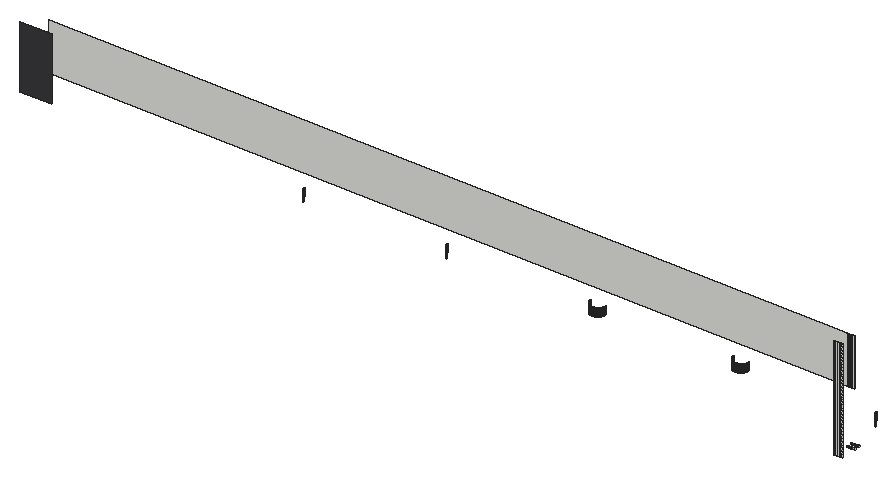
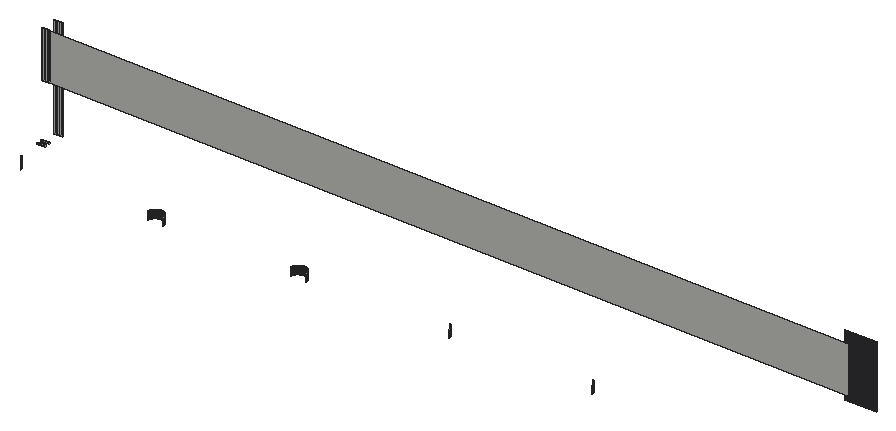
# SketchUp Ruby script. Lengths in inches.
U = 1.inch
M = Sketchup.active_model
def pt(a) = Geom::Point3d.new(a.map { |v| v * U })
def face(e, loops, mat)
  f = e.add_face(loops[0].map { |a| pt(a) })
  loops[1..].each { |l| e.add_face(l.map { |a| pt(a) }).erase! }
  f.material = f.back_material = mat if mat
  f
end
# faces: each face lists its corners as indices into pts; further lists are holes
def faces(e, pts, list, mat = nil) = list.each { |f| face(e, (f[0].is_a?(Array) ? f : [f]).map { |l| l.map { |i| pts[i] } }, mat) }
# xy, xz, yz: faces in a plane at the given z, y or x. An outline is a flat list of corners, or four numbers for a rectangle; further outlines are holes
def ring(l) = l.size == 4 ? [[l[0], l[1]], [l[2], l[1]], [l[2], l[3]], [l[0], l[3]]] : l.each_slice(2).to_a
def flat(e, list, mat, &to3) = list.each { |f| face(e, (f[0].is_a?(Array) ? f : [f]).map { |l| ring(l).map { |u, v| to3.(u, v) } }, mat) }
def xy(e, z, list, mat = nil) = flat(e, list, mat) { |x, y| [x, y, z] }
def xz(e, y, list, mat = nil) = flat(e, list, mat) { |x, z| [x, y, z] }
def yz(e, x, list, mat = nil) = flat(e, list, mat) { |y, z| [x, y, z] }
def lines(e, pts, list) = list.each { |a, b| e.add_line(pt(pts[a]), pt(pts[b])) }
# prism: a flat outline (further loops are holes) pulled along v
def prism(e, loops, v, mat = nil)
  f = face(e, loops, mat); d = Geom::Vector3d.new(v.map { |x| x * U })
  f.pushpull(f.normal.samedirection?(d) ? d.length : -d.length)
end
def box(e, o, s, mat = nil) = prism(e, [[o, [o[0] + s[0], o[1], o[2]], [o[0] + s[0], o[1] + s[1], o[2]], [o[0], o[1] + s[1], o[2]]]], [0, 0, s[2]], mat)
def at(x, y, z, deg = 0) = Geom::Transformation.translation(pt([x, y, z])) * Geom::Transformation.rotation(ORIGIN, Z_AXIS, deg.degrees)
def axes(o, x, y, z) = Geom::Transformation.new([*x, 0, *y, 0, *z, 0, *pt(o).to_a, 1])
def part(name) = M.definitions.add(name)
# library, detail: a bought-in or finely detailed component or shape, given as its bounding box
def library(name, o, s) = part(name).tap { |d| box(d.entities, o, s) }
def detail(e, o, s) = box(e.add_group.entities, o, s)
def put(e, d, t, mat = nil) = e.add_instance(d, t).tap { |i| i.material = mat if mat }
def group(e, t, mat = nil) = e.add_group.tap { |g| g.transformation = t; g.material = mat if mat }.entities
root = M.entities
M.materials.add("1432 AP 8245 TAR ROAD").color = [57, 57, 60]
xz(root,164,[[324,231,324.3125,270]])
xz(root,164,[[12,246,24,270]],"1432 AP 8245 TAR ROAD")
xz(root,170,[[324,231,324.24,231.5],[18,252,324,270],[324,252,324.24,270]])
xz(root,170.01,[[324.47,231,324.71,231.5],[324.47,252,324.71,270]])
xz(root,172,[[324,231,324.21,231.5]])
xz(root,172.01,[[324.42,231,324.63,231.5]])
xz(root,185,[[214.28,231,214.35,234],[214.35,231,214.43,234],[214.43,231,214.51,234],[269.08,231,269.15,234],[269.15,231,269.23,234],
  [269.23,231,269.3125,234]])
xz(root,185.01,[[214.12,231,214.2,234],[214.59,231,214.67,234],[268.92,231,269,234],[269.39,231,269.47,234]])
yz(root,156.61,[[187.73,231,187.81,234]])
yz(root,211.41,[[187.73,231,187.81,234]])
yz(root,217.39,[[187.72,231,187.8,234]])
yz(root,266.21,[[187.73,231,187.81,234]])
yz(root,321.01,[[187.73,231,187.81,234]])
p = [[324.63,164.01,231],[324.63,164.01,270],[324.3125,164,270],[324.3125,164,231],[324.94,164.02,231],[324.94,164.02,270],
  [325.26,164.03,231],[325.26,164.03,270],[325.57,164.05,231],[325.57,164.05,270],[325.88,164.07,231],[325.88,164.07,270],
  [326.2,164.1,231],[326.2,164.1,270],[326.51,164.13,231],[326.51,164.13,270],[326.82,164.17,231],[326.82,164.17,270],
  [327.13,164.21,231],[327.13,164.21,270],[324.47,170.01,231],[324.24,170,231],[324.24,170,231.5],[324.47,170.01,231.5],
  [324.94,170.02,231],[324.71,170.01,231],[324.71,170.01,231.5],[324.94,170.02,231.5],[325.18,170.04,231],[325.18,170.04,231.5],
  [325.41,170.06,231],[325.41,170.06,231.5],[325.65,170.08,231],[325.65,170.08,231.5],[325.88,170.1,231],[325.88,170.1,231.5],
  [326.12,170.125,231],[326.12,170.125,231.5],[326.35,170.15,231],[326.35,170.15,231.5],[326.58,170.1875,231],[326.58,170.1875,231.5],
  [326.82,170.22,231],[326.82,170.22,231.5],[327.05,170.26,231],[327.05,170.26,231.5],[327.28,170.3,231],[327.28,170.3,231.5],
  [324.21,172,231],[324.42,172.01,231],[324.42,172.01,231.5],[324.21,172,231.5],[324.63,172.01,231],[324.84,172.02,231],
  [324.84,172.02,231.5],[324.63,172.01,231.5],[325.05,172.03,231],[325.05,172.03,231.5],[325.26,172.05,231],[325.26,172.05,231.5],
  [325.46,172.07,231],[325.46,172.07,231.5],[325.67,172.09,231],[325.67,172.09,231.5],[325.88,172.11,231],[325.88,172.11,231.5],
  [326.09,172.14,231],[326.09,172.14,231.5],[326.3,172.17,231],[326.3,172.17,231.5],[326.5,172.2,231],[326.5,172.2,231.5],
  [326.71,172.23,231],[326.71,172.23,231.5],[326.92,172.27,231],[326.92,172.27,231.5],[327.12,172.31,231],[327.12,172.31,231.5],
  [213.89,185.04,231],[213.81,185.06,231],[213.81,185.06,234],[213.89,185.04,234],[213.96,185.03,231],[213.96,185.03,234],
  [214.04,185.02,231],[214.04,185.02,234],[214.12,185.01,231],[214.12,185.01,234],[214.28,185,231],[214.2,185.01,231],
  [214.2,185.01,234],[214.28,185,234],[214.59,185.01,231],[214.51,185,231],[214.51,185,234],[214.59,185.01,234],
  [214.75,185.02,231],[214.67,185.01,231],[214.67,185.01,234],[214.75,185.02,234],[214.82,185.03,231],[214.82,185.03,234],
  [214.9,185.04,231],[214.9,185.04,234],[214.98,185.06,231],[214.98,185.06,234],[268.6875,185.04,231],[268.61,185.06,231],
  [268.61,185.06,234],[268.6875,185.04,234],[268.76,185.03,231],[268.76,185.03,234],[268.84,185.02,231],[268.84,185.02,234],
  [268.92,185.01,231],[268.92,185.01,234],[269.08,185,231],[269,185.01,231],[269,185.01,234],[269.08,185,234],
  [269.39,185.01,231],[269.3125,185,231],[269.3125,185,234],[269.39,185.01,234],[269.55,185.02,231],[269.47,185.01,231],
  [269.47,185.01,234],[269.55,185.02,234],[269.625,185.03,231],[269.625,185.03,234],[269.7,185.04,231],[269.7,185.04,234],
  [269.78,185.06,231],[269.78,185.06,234],[103.9,185.14,231],[103.83,185.16,231],[103.83,185.16,234],[103.9,185.14,234],
  [158.7,185.14,231],[158.63,185.16,231],[158.63,185.16,234],[158.7,185.14,234],[213.5,185.14,231],[213.43,185.16,231],
  [213.43,185.16,234],[213.5,185.14,234],[213.58,185.11,231],[213.58,185.11,234],[213.66,185.09,231],[213.66,185.09,234],
  [213.73,185.08,231],[213.73,185.08,234],[215.06,185.07,231],[215.06,185.07,234],[215.13,185.09,231],[215.13,185.09,234],
  [215.21,185.11,231],[215.21,185.11,234],[215.28,185.13,231],[215.28,185.13,234],[215.36,185.16,231],[215.36,185.16,234],
  [268.3,185.14,231],[268.23,185.16,231],[268.23,185.16,234],[268.3,185.14,234],[268.38,185.11,231],[268.38,185.11,234],
  [268.46,185.09,231],[268.46,185.09,234],[268.53,185.08,231],[268.53,185.08,234],[269.86,185.07,231],[269.86,185.07,234],
  [269.93,185.09,231],[269.93,185.09,234],[270.01,185.11,231],[270.01,185.11,234],[270.08,185.13,231],[270.08,185.13,234],
  [270.16,185.16,231],[270.16,185.16,234],[323.1,185.14,231],[323.03,185.16,231],[323.03,185.16,234],[323.1,185.14,234],
  [103.61,185.25,231],[103.54,185.28,231],[103.54,185.28,234],[103.61,185.25,234],[103.68,185.22,231],[103.68,185.22,234],
  [103.76,185.1875,231],[103.76,185.1875,234],[158.41,185.25,231],[158.34,185.28,231],[158.34,185.28,234],[158.41,185.25,234],
  [158.48,185.22,231],[158.48,185.22,234],[158.56,185.1875,231],[158.56,185.1875,234],[213.21,185.25,231],[213.14,185.28,231],
  [213.14,185.28,234],[213.21,185.25,234],[213.28,185.22,231],[213.28,185.22,234],[213.36,185.1875,231],[213.36,185.1875,234],
  [215.43,185.18,231],[215.43,185.18,234],[215.51,185.21,231],[215.51,185.21,234],[215.58,185.24,231],[215.58,185.24,234],
  [215.65,185.27,231],[215.65,185.27,234],[268.01,185.25,231],[267.9375,185.28,231],[267.9375,185.28,234],[268.01,185.25,234],
  [268.08,185.22,231],[268.08,185.22,234],[268.16,185.1875,231],[268.16,185.1875,234],[270.23,185.18,231],[270.23,185.18,234],
  [270.31,185.21,231],[270.31,185.21,234],[270.38,185.24,231],[270.38,185.24,234],[270.45,185.27,231],[270.45,185.27,234],
  [322.81,185.25,231],[322.74,185.28,231],[322.74,185.28,234],[322.81,185.25,234],[322.88,185.22,231],[322.88,185.22,234],
  [322.96,185.1875,231],[322.96,185.1875,234],[103.4,185.35,231],[103.33,185.39,231],[103.33,185.39,234],[103.4,185.35,234],
  [103.47,185.3125,231],[103.47,185.3125,234],[158.2,185.35,231],[158.13,185.39,231],[158.13,185.39,234],[158.2,185.35,234],
  [158.27,185.3125,231],[158.27,185.3125,234],[213,185.35,231],[212.93,185.39,231],[212.93,185.39,234],[213,185.35,234],
  [213.07,185.3125,231],[213.07,185.3125,234],[215.72,185.31,231],[215.72,185.31,234],[215.79,185.34,231],[215.79,185.34,234],
  [215.86,185.38,231],[215.86,185.38,234],[267.8,185.35,231],[267.73,185.39,231],[267.73,185.39,234],[267.8,185.35,234],
  [267.87,185.3125,231],[267.87,185.3125,234],[270.52,185.31,231],[270.52,185.31,234],[270.59,185.34,231],[270.59,185.34,234],
  [270.66,185.38,231],[270.66,185.38,234],[322.6,185.35,231],[322.53,185.39,231],[322.53,185.39,234],[322.6,185.35,234],
  [322.67,185.3125,231],[322.67,185.3125,234],[103.26,185.42,231],[103.19,185.47,231],[103.19,185.47,234],[103.26,185.42,234],
  [158.0625,185.42,231],[157.99,185.47,231],[157.99,185.47,234],[158.0625,185.42,234],[212.86,185.42,231],[212.79,185.47,231],
  [212.79,185.47,234],[212.86,185.42,234],[215.93,185.42,231],[215.93,185.42,234],[216,185.46,231],[216,185.46,234],
  [267.66,185.42,231],[267.59,185.47,231],[267.59,185.47,234],[267.66,185.42,234],[270.73,185.42,231],[270.73,185.42,234],
  [270.8,185.46,231],[270.8,185.46,234],[322.46,185.42,231],[322.39,185.47,231],[322.39,185.47,234],[322.46,185.42,234],
  [103.13,185.51,231],[103.0625,185.55,231],[103.0625,185.55,234],[103.13,185.51,234],[157.93,185.51,231],[157.86,185.55,231],
  [157.86,185.55,234],[157.93,185.51,234],[212.73,185.51,231],[212.66,185.55,231],[212.66,185.55,234],[212.73,185.51,234],
  [216.0625,185.5,231],[216.0625,185.5,234],[216.125,185.55,231],[216.125,185.55,234],[216.19,185.59,231],[216.19,185.59,234],
  [267.53,185.51,231],[267.46,185.55,231],[267.46,185.55,234],[267.53,185.51,234],[270.86,185.5,231],[270.86,185.5,234],
  [270.93,185.55,231],[270.93,185.55,234],[270.99,185.59,231],[270.99,185.59,234],[322.33,185.51,231],[322.26,185.55,231],
  [322.26,185.55,234],[322.33,185.51,234],[102.9375,185.65,231],[102.88,185.7,231],[102.88,185.7,234],[102.9375,185.65,234],
  [103,185.6,231],[103,185.6,234],[157.74,185.65,231],[157.68,185.7,231],[157.68,185.7,234],[157.74,185.65,234],
  [157.8,185.6,231],[157.8,185.6,234],[212.54,185.65,231],[212.48,185.7,231],[212.48,185.7,234],[212.54,185.65,234],
  [212.6,185.6,231],[212.6,185.6,234],[216.25,185.64,231],[216.25,185.64,234],[216.3125,185.69,231],[216.3125,185.69,234],
  [267.34,185.65,231],[267.28,185.7,231],[267.28,185.7,234],[267.34,185.65,234],[267.4,185.6,231],[267.4,185.6,234],
  [271.05,185.64,231],[271.05,185.64,234],[271.11,185.69,231],[271.11,185.69,234],[322.14,185.65,231],[322.08,185.7,231],
  [322.08,185.7,234],[322.14,185.65,234],[322.2,185.6,231],[322.2,185.6,234],[102.82,185.75,231],[102.76,185.8,231],
  [102.76,185.8,234],[102.82,185.75,234],[157.62,185.75,231],[157.56,185.8,231],[157.56,185.8,234],[157.62,185.75,234],
  [212.42,185.75,231],[212.36,185.8,231],[212.36,185.8,234],[212.42,185.75,234],[216.375,185.74,231],[216.375,185.74,234],
  [216.43,185.79,231],[216.43,185.79,234],[267.22,185.75,231],[267.16,185.8,231],[267.16,185.8,234],[267.22,185.75,234],
  [271.17,185.74,231],[271.17,185.74,234],[271.23,185.79,231],[271.23,185.79,234],[322.02,185.75,231],[321.96,185.8,231],
  [321.96,185.8,234],[322.02,185.75,234],[102.7,185.86,231],[102.7,185.86,234],[157.5,185.86,231],[157.5,185.86,234],
  [212.3,185.86,231],[212.3,185.86,234],[216.49,185.85,231],[216.49,185.85,234],[216.54,185.9,231],[216.54,185.9,234],
  [267.1,185.86,231],[267.1,185.86,234],[271.29,185.85,231],[271.29,185.85,234],[271.34,185.9,231],[271.34,185.9,234],
  [321.9,185.86,231],[321.9,185.86,234],[102.65,185.91,231],[102.59,185.97,231],[102.59,185.97,234],[102.65,185.91,234],
  [157.45,185.91,231],[157.39,185.97,231],[157.39,185.97,234],[157.45,185.91,234],[212.25,185.91,231],[212.19,185.97,231],
  [212.19,185.97,234],[212.25,185.91,234],[216.6,185.96,231],[216.6,185.96,234],[267.05,185.91,231],[266.99,185.97,231],
  [266.99,185.97,234],[267.05,185.91,234],[271.4,185.96,231],[271.4,185.96,234],[321.85,185.91,231],[321.79,185.97,231],
  [321.79,185.97,234],[321.85,185.91,234],[102.54,186.03,231],[102.49,186.09,231],[102.49,186.09,234],[102.54,186.03,234],
  [157.34,186.03,231],[157.29,186.09,231],[157.29,186.09,234],[157.34,186.03,234],[212.14,186.03,231],[212.09,186.09,231],
  [212.09,186.09,234],[212.14,186.03,234],[216.65,186.02,231],[216.65,186.02,234],[216.7,186.08,231],[216.7,186.08,234],
  [266.94,186.03,231],[266.89,186.09,231],[266.89,186.09,234],[266.94,186.03,234],[271.45,186.02,231],[271.45,186.02,234],
  [271.5,186.08,231],[271.5,186.08,234],[321.74,186.03,231],[321.69,186.09,231],[321.69,186.09,234],[321.74,186.03,234],
  [102.44,186.15,231],[102.39,186.21,231],[102.39,186.21,234],[102.44,186.15,234],[157.24,186.15,231],[157.19,186.21,231],
  [157.19,186.21,234],[157.24,186.15,234],[212.04,186.15,231],[211.99,186.21,231],[211.99,186.21,234],[212.04,186.15,234],
  [216.75,186.14,231],[216.75,186.14,234],[216.8,186.2,231],[216.8,186.2,234],[266.84,186.15,231],[266.79,186.21,231],
  [266.79,186.21,234],[266.84,186.15,234],[271.55,186.14,231],[271.55,186.14,234],[271.6,186.2,231],[271.6,186.2,234],
  [321.64,186.15,231],[321.59,186.21,231],[321.59,186.21,234],[321.64,186.15,234],[102.35,186.27,231],[102.35,186.27,234],
  [157.15,186.27,231],[157.15,186.27,234],[211.95,186.27,231],[211.95,186.27,234],[216.85,186.26,231],[216.85,186.26,234],
  [266.75,186.27,231],[266.75,186.27,234],[271.65,186.26,231],[271.65,186.26,234],[321.55,186.27,231],[321.55,186.27,234],
  [102.3,186.34,231],[102.26,186.4,231],[102.26,186.4,234],[102.3,186.34,234],[157.1,186.34,231],[157.06,186.4,231],
  [157.06,186.4,234],[157.1,186.34,234],[211.9,186.34,231],[211.86,186.4,231],[211.86,186.4,234],[211.9,186.34,234],
  [216.89,186.33,231],[216.89,186.33,234],[216.93,186.39,231],[216.93,186.39,234],[266.7,186.34,231],[266.66,186.4,231],
  [266.66,186.4,234],[266.7,186.34,234],[271.69,186.33,231],[271.69,186.33,234],[271.73,186.39,231],[271.73,186.39,234],
  [321.5,186.34,231],[321.46,186.4,231],[321.46,186.4,234],[321.5,186.34,234],[102.22,186.47,231],[102.22,186.47,234],
  [157.02,186.47,231],[157.02,186.47,234],[211.82,186.47,231],[211.82,186.47,234],[216.98,186.46,231],[216.98,186.46,234],
  [266.62,186.47,231],[266.62,186.47,234],[271.78,186.46,231],[271.78,186.46,234],[321.42,186.47,231],[321.42,186.47,234],
  [102.18,186.54,231],[102.14,186.61,231],[102.14,186.61,234],[102.18,186.54,234],[156.98,186.54,231],[156.94,186.61,231],
  [156.94,186.61,234],[156.98,186.54,234],[211.78,186.54,231],[211.74,186.61,231],[211.74,186.61,234],[211.78,186.54,234],
  [217.01,186.53,231],[217.01,186.53,234],[217.05,186.6,231],[217.05,186.6,234],[266.58,186.54,231],[266.54,186.61,231],
  [266.54,186.61,234],[266.58,186.54,234],[271.81,186.53,231],[271.81,186.53,234],[271.85,186.6,231],[271.85,186.6,234],
  [321.38,186.54,231],[321.34,186.61,231],[321.34,186.61,234],[321.38,186.54,234],[102.11,186.68,231],[102.11,186.68,234],
  [156.91,186.68,231],[156.91,186.68,234],[211.71,186.68,231],[211.71,186.68,234],[217.09,186.67,231],[217.09,186.67,234],
  [266.51,186.68,231],[266.51,186.68,234],[271.89,186.67,231],[271.89,186.67,234],[321.31,186.68,231],[321.31,186.68,234],
  [102.07,186.75,231],[102.04,186.82,231],[102.04,186.82,234],[102.07,186.75,234],[156.875,186.75,231],[156.84,186.82,231],
  [156.84,186.82,234],[156.875,186.75,234],[211.67,186.75,231],[211.64,186.82,231],[211.64,186.82,234],[211.67,186.75,234],
  [217.12,186.74,231],[217.12,186.74,234],[217.15,186.81,231],[217.15,186.81,234],[266.47,186.75,231],[266.44,186.82,231],
  [266.44,186.82,234],[266.47,186.75,234],[271.92,186.74,231],[271.92,186.74,234],[271.95,186.81,231],[271.95,186.81,234],
  [321.27,186.75,231],[321.24,186.82,231],[321.24,186.82,234],[321.27,186.75,234],[102.01,186.89,231],[102.01,186.89,234],
  [156.8125,186.89,231],[156.8125,186.89,234],[211.61,186.89,231],[211.61,186.89,234],[217.18,186.88,231],[217.18,186.88,234],
  [266.41,186.89,231],[266.41,186.89,234],[271.98,186.88,231],[271.98,186.88,234],[321.21,186.89,231],[321.21,186.89,234],
  [101.98,186.97,231],[101.98,186.97,234],[156.78,186.97,231],[156.78,186.97,234],[211.58,186.97,231],[211.58,186.97,234],
  [217.21,186.96,231],[217.21,186.96,234],[266.38,186.97,231],[266.38,186.97,234],[272.01,186.96,231],[272.01,186.96,234],
  [321.18,186.97,231],[321.18,186.97,234],[101.96,187.04,231],[101.93,187.12,231],[101.93,187.12,234],[101.96,187.04,234],
  [156.76,187.04,231],[156.73,187.12,231],[156.73,187.12,234],[156.76,187.04,234],[211.56,187.04,231],[211.53,187.12,231],
  [211.53,187.12,234],[211.56,187.04,234],[217.24,187.03,231],[217.24,187.03,234],[217.26,187.1,231],[217.26,187.1,234],
  [266.36,187.04,231],[266.33,187.12,231],[266.33,187.12,234],[266.36,187.04,234],[272.04,187.03,231],[272.04,187.03,234],
  [272.0625,187.1,231],[272.0625,187.1,234],[321.16,187.04,231],[321.13,187.12,231],[321.13,187.12,234],[321.16,187.04,234],
  [101.91,187.19,231],[101.91,187.19,234],[156.71,187.19,231],[156.71,187.19,234],[211.51,187.19,231],[211.51,187.19,234],
  [217.29,187.18,231],[217.29,187.18,234],[266.3125,187.19,231],[266.3125,187.19,234],[272.09,187.18,231],[272.09,187.18,234],
  [321.11,187.19,231],[321.11,187.19,234],[101.89,187.27,231],[101.89,187.27,234],[156.69,187.27,231],[156.69,187.27,234],
  [211.49,187.27,231],[211.49,187.27,234],[217.31,187.26,231],[217.31,187.26,234],[266.29,187.27,231],[266.29,187.27,234],
  [272.11,187.26,231],[272.11,187.26,234],[321.09,187.27,231],[321.09,187.27,234],[101.87,187.34,231],[101.86,187.42,231],
  [101.86,187.42,234],[101.87,187.34,234],[156.67,187.34,231],[156.66,187.42,231],[156.66,187.42,234],[156.67,187.34,234],
  [211.47,187.34,231],[211.46,187.42,231],[211.46,187.42,234],[211.47,187.34,234],[217.32,187.33,231],[217.32,187.33,234],
  [217.34,187.41,231],[217.34,187.41,234],[266.27,187.34,231],[266.26,187.42,231],[266.26,187.42,234],[266.27,187.34,234],
  [272.125,187.33,231],[272.125,187.33,234],[272.14,187.41,231],[272.14,187.41,234],[321.07,187.34,231],[321.06,187.42,231],
  [321.06,187.42,234],[321.07,187.34,234],[101.84,187.5,231],[101.84,187.5,234],[156.64,187.5,231],[156.64,187.5,234],
  [211.44,187.5,231],[211.44,187.5,234],[217.36,187.49,231],[217.36,187.49,234],[266.24,187.5,231],[266.24,187.5,234],
  [272.16,187.49,231],[272.16,187.49,234],[321.04,187.5,231],[321.04,187.5,234],[101.83,187.58,231],[101.83,187.58,234],
  [156.63,187.58,231],[156.63,187.58,234],[211.43,187.58,231],[211.43,187.58,234],[217.37,187.5625,231],[217.37,187.5625,234],
  [266.23,187.58,231],[266.23,187.58,234],[272.17,187.5625,231],[272.17,187.5625,234],[321.03,187.58,231],[321.03,187.58,234],
  [101.82,187.65,231],[101.82,187.65,234],[156.62,187.65,231],[156.62,187.65,234],[211.42,187.65,231],[211.42,187.65,234],
  [217.38,187.64,231],[217.38,187.64,234],[217.39,187.72,231],[217.39,187.72,234],[266.22,187.65,231],[266.22,187.65,234],
  [272.18,187.64,231],[272.18,187.64,234],[272.1875,187.72,231],[272.1875,187.72,234],[321.02,187.65,231],[321.02,187.65,234],
  [101.8125,187.73,231],[101.81,187.81,231],[101.81,187.81,234],[101.8125,187.73,234],[156.61,187.73,231],[156.61,187.73,234],
  [211.41,187.73,231],[211.41,187.73,234],[266.21,187.73,231],[266.21,187.73,234],[272.19,187.8,231],[272.19,187.8,234],
  [321.01,187.73,231],[321.01,187.73,234],[101.8,187.89,231],[101.8,187.89,234],[156.61,187.81,231],[156.6,187.89,231],
  [156.6,187.89,234],[156.61,187.81,234],[211.41,187.81,231],[211.4,187.89,231],[211.4,187.89,234],[211.41,187.81,234],
  [217.4,187.875,231],[217.39,187.8,231],[217.39,187.8,234],[217.4,187.875,234],[266.21,187.81,231],[266.2,187.89,231],
  [266.2,187.89,234],[266.21,187.81,234],[272.2,187.875,231],[272.2,187.875,234],[321.01,187.81,231],[321,187.89,231],
  [321,187.89,234],[321.01,187.81,234],[324.47,170.01,252],[324.24,170,252],[324.24,170,270],[324.47,170.01,270],
  [324.94,170.02,252],[324.71,170.01,252],[324.71,170.01,270],[324.94,170.02,270],[325.18,170.04,252],[325.18,170.04,270],
  [325.41,170.06,252],[325.41,170.06,270],[325.65,170.08,252],[325.65,170.08,270],[325.88,170.1,252],[325.88,170.1,270],
  [326.12,170.125,252],[326.12,170.125,270],[326.35,170.15,252],[326.35,170.15,270],[326.58,170.1875,252],[326.58,170.1875,270],
  [326.82,170.22,252],[326.82,170.22,270],[327.05,170.26,252],[327.05,170.26,270]]
faces(root,p,[[0,1,2,3],[4,5,1,0],[6,7,5,4],[8,9,7,6],[10,11,9,8],[12,13,11,10],[14,15,13,12],[16,17,15,14],
  [18,19,17,16],[20,21,22,23],[24,25,26,27],[28,24,27,29],[30,28,29,31],[32,30,31,33],[34,32,33,35],[36,34,35,37],
  [38,36,37,39],[40,38,39,41],[42,40,41,43],[44,42,43,45],[46,44,45,47],[48,49,50,51],[52,53,54,55],[53,56,57,54],
  [56,58,59,57],[58,60,61,59],[60,62,63,61],[62,64,65,63],[64,66,67,65],[66,68,69,67],[68,70,71,69],[70,72,73,71],
  [72,74,75,73],[74,76,77,75],[78,79,80,81],[82,78,81,83],[84,82,83,85],[86,84,85,87],[88,89,90,91],[92,93,94,95],
  [96,97,98,99],[100,96,99,101],[102,100,101,103],[104,102,103,105],[106,107,108,109],[110,106,109,111],[112,110,111,113],[114,112,113,115],
  [116,117,118,119],[120,121,122,123],[124,125,126,127],[128,124,127,129],[130,128,129,131],[132,130,131,133],[134,135,136,137],[138,139,140,141],
  [142,143,144,145],[146,142,145,147],[148,146,147,149],[150,148,149,151],[79,150,151,80],[152,104,105,153],[154,152,153,155],[156,154,155,157],
  [158,156,157,159],[160,158,159,161],[162,163,164,165],[166,162,165,167],[168,166,167,169],[170,168,169,171],[107,170,171,108],[172,132,133,173],
  [174,172,173,175],[176,174,175,177],[178,176,177,179],[180,178,179,181],[182,183,184,185],[186,187,188,189],[190,186,189,191],[192,190,191,193],
  [135,192,193,136],[194,195,196,197],[198,194,197,199],[200,198,199,201],[139,200,201,140],[202,203,204,205],[206,202,205,207],[208,206,207,209],
  [143,208,209,144],[210,160,161,211],[212,210,211,213],[214,212,213,215],[216,214,215,217],[218,219,220,221],[222,218,221,223],[224,222,223,225],
  [163,224,225,164],[226,180,181,227],[228,226,227,229],[230,228,229,231],[232,230,231,233],[234,235,236,237],[238,234,237,239],[240,238,239,241],
  [183,240,241,184],[242,243,244,245],[246,242,245,247],[187,246,247,188],[248,249,250,251],[252,248,251,253],[195,252,253,196],[254,255,256,257],
  [258,254,257,259],[203,258,259,204],[260,216,217,261],[262,260,261,263],[264,262,263,265],[266,267,268,269],[270,266,269,271],[219,270,271,220],
  [272,232,233,273],[274,272,273,275],[276,274,275,277],[278,279,280,281],[282,278,281,283],[235,282,283,236],[284,285,286,287],[243,284,287,244],
  [288,289,290,291],[249,288,291,250],[292,293,294,295],[255,292,295,256],[296,264,265,297],[298,296,297,299],[300,301,302,303],[267,300,303,268],
  [304,276,277,305],[306,304,305,307],[308,309,310,311],[279,308,311,280],[312,313,314,315],[285,312,315,286],[316,317,318,319],[289,316,319,290],
  [320,321,322,323],[293,320,323,294],[324,298,299,325],[326,324,325,327],[328,326,327,329],[330,331,332,333],[301,330,333,302],[334,306,307,335],
  [336,334,335,337],[338,336,337,339],[340,341,342,343],[309,340,343,310],[344,345,346,347],[348,344,347,349],[313,348,349,314],[350,351,352,353],
  [354,350,353,355],[317,354,355,318],[356,357,358,359],[360,356,359,361],[321,360,361,322],[362,328,329,363],[364,362,363,365],[366,367,368,369],
  [370,366,369,371],[331,370,371,332],[372,338,339,373],[374,372,373,375],[376,377,378,379],[380,376,379,381],[341,380,381,342],[382,383,384,385],
  [345,382,385,346],[386,387,388,389],[351,386,389,352],[390,391,392,393],[357,390,393,358],[394,364,365,395],[396,394,395,397],[398,399,400,401],
  [367,398,401,368],[402,374,375,403],[404,402,403,405],[406,407,408,409],[377,406,409,378],[383,410,411,384],[387,412,413,388],[391,414,415,392],
  [416,396,397,417],[418,416,417,419],[399,420,421,400],[422,404,405,423],[424,422,423,425],[407,426,427,408],[428,429,430,431],[410,428,431,411],
  [432,433,434,435],[412,432,435,413],[436,437,438,439],[414,436,439,415],[440,418,419,441],[442,443,444,445],[420,442,445,421],[446,424,425,447],
  [448,449,450,451],[426,448,451,427],[452,453,454,455],[429,452,455,430],[456,457,458,459],[433,456,459,434],[460,461,462,463],[437,460,463,438],
  [464,440,441,465],[466,464,465,467],[468,469,470,471],[443,468,471,444],[472,446,447,473],[474,472,473,475],[476,477,478,479],[449,476,479,450],
  [480,481,482,483],[453,480,483,454],[484,485,486,487],[457,484,487,458],[488,489,490,491],[461,488,491,462],[492,466,467,493],[494,492,493,495],
  [496,497,498,499],[469,496,499,470],[500,474,475,501],[502,500,501,503],[504,505,506,507],[477,504,507,478],[481,508,509,482],[485,510,511,486],
  [489,512,513,490],[514,494,495,515],[497,516,517,498],[518,502,503,519],[505,520,521,506],[522,523,524,525],[508,522,525,509],[526,527,528,529],
  [510,526,529,511],[530,531,532,533],[512,530,533,513],[534,514,515,535],[536,534,535,537],[538,539,540,541],[516,538,541,517],[542,518,519,543],
  [544,542,543,545],[546,547,548,549],[520,546,549,521],[523,550,551,524],[527,552,553,528],[531,554,555,532],[556,536,537,557],[539,558,559,540],
  [560,544,545,561],[547,562,563,548],[564,565,566,567],[550,564,567,551],[568,569,570,571],[552,568,571,553],[572,573,574,575],[554,572,575,555],
  [576,556,557,577],[578,576,577,579],[580,581,582,583],[558,580,583,559],[584,560,561,585],[586,584,585,587],[588,589,590,591],[562,588,591,563],
  [565,592,593,566],[569,594,595,570],[573,596,597,574],[598,578,579,599],[581,600,601,582],[602,586,587,603],[589,604,605,590],[606,607,608,609],
  [592,606,609,593],[610,611,612,613],[594,610,613,595],[614,615,616,617],[596,614,617,597],[618,598,599,619],[620,618,619,621],[622,623,624,625],
  [600,622,625,601],[626,602,603,627],[628,626,627,629],[630,631,632,633],[604,630,633,605],[607,634,635,608],[611,636,637,612],[615,638,639,616],
  [640,620,621,641],[623,642,643,624],[644,628,629,645],[631,646,647,632],[634,648,649,635],[636,650,651,637],[638,652,653,639],[654,640,641,655],
  [642,656,657,643],[658,644,645,659],[646,660,661,647],[662,663,664,665],[648,662,665,649],[666,667,668,669],[650,666,669,651],[670,671,672,673],
  [652,670,673,653],[674,654,655,675],[676,674,675,677],[678,679,680,681],[656,678,681,657],[682,658,659,683],[684,682,683,685],[686,687,688,689],
  [660,686,689,661],[663,690,691,664],[667,692,693,668],[671,694,695,672],[696,676,677,697],[679,698,699,680],[700,684,685,701],[687,702,703,688],
  [690,704,705,691],[692,706,707,693],[694,708,709,695],[710,696,697,711],[698,712,713,699],[714,700,701,715],[702,716,717,703],[718,719,720,721],
  [704,718,721,705],[722,723,724,725],[706,722,725,707],[726,727,728,729],[708,726,729,709],[730,710,711,731],[732,730,731,733],[734,735,736,737],
  [712,734,737,713],[738,714,715,739],[740,738,739,741],[742,743,744,745],[716,742,745,717],[719,746,747,720],[723,748,749,724],[727,750,751,728],
  [752,732,733,753],[735,754,755,736],[756,740,741,757],[743,758,759,744],[746,760,761,747],[748,762,763,749],[750,764,765,751],[766,752,753,767],
  [754,768,769,755],[770,756,757,771],[758,772,773,759],[760,774,775,761],[762,776,777,763],[764,778,779,765],[780,766,767,781],[782,780,781,783],
  [768,784,785,769],[786,770,771,787],[788,786,787,789],[772,790,791,773],[792,793,794,795],[774,792,795,775],[776,796,797,777],[778,798,799,779],
  [784,800,801,785],[802,788,789,803],[790,804,805,791],[793,806,807,794],[808,809,810,811],[812,813,814,815],[816,817,818,819],[820,821,822,823],
  [824,802,803,825],[826,827,828,829],[830,831,832,833],[834,835,836,837],[838,834,837,839],[840,838,839,841],[842,840,841,843],[844,842,843,845],
  [846,844,845,847],[848,846,847,849],[850,848,849,851],[852,850,851,853],[854,852,853,855]])
